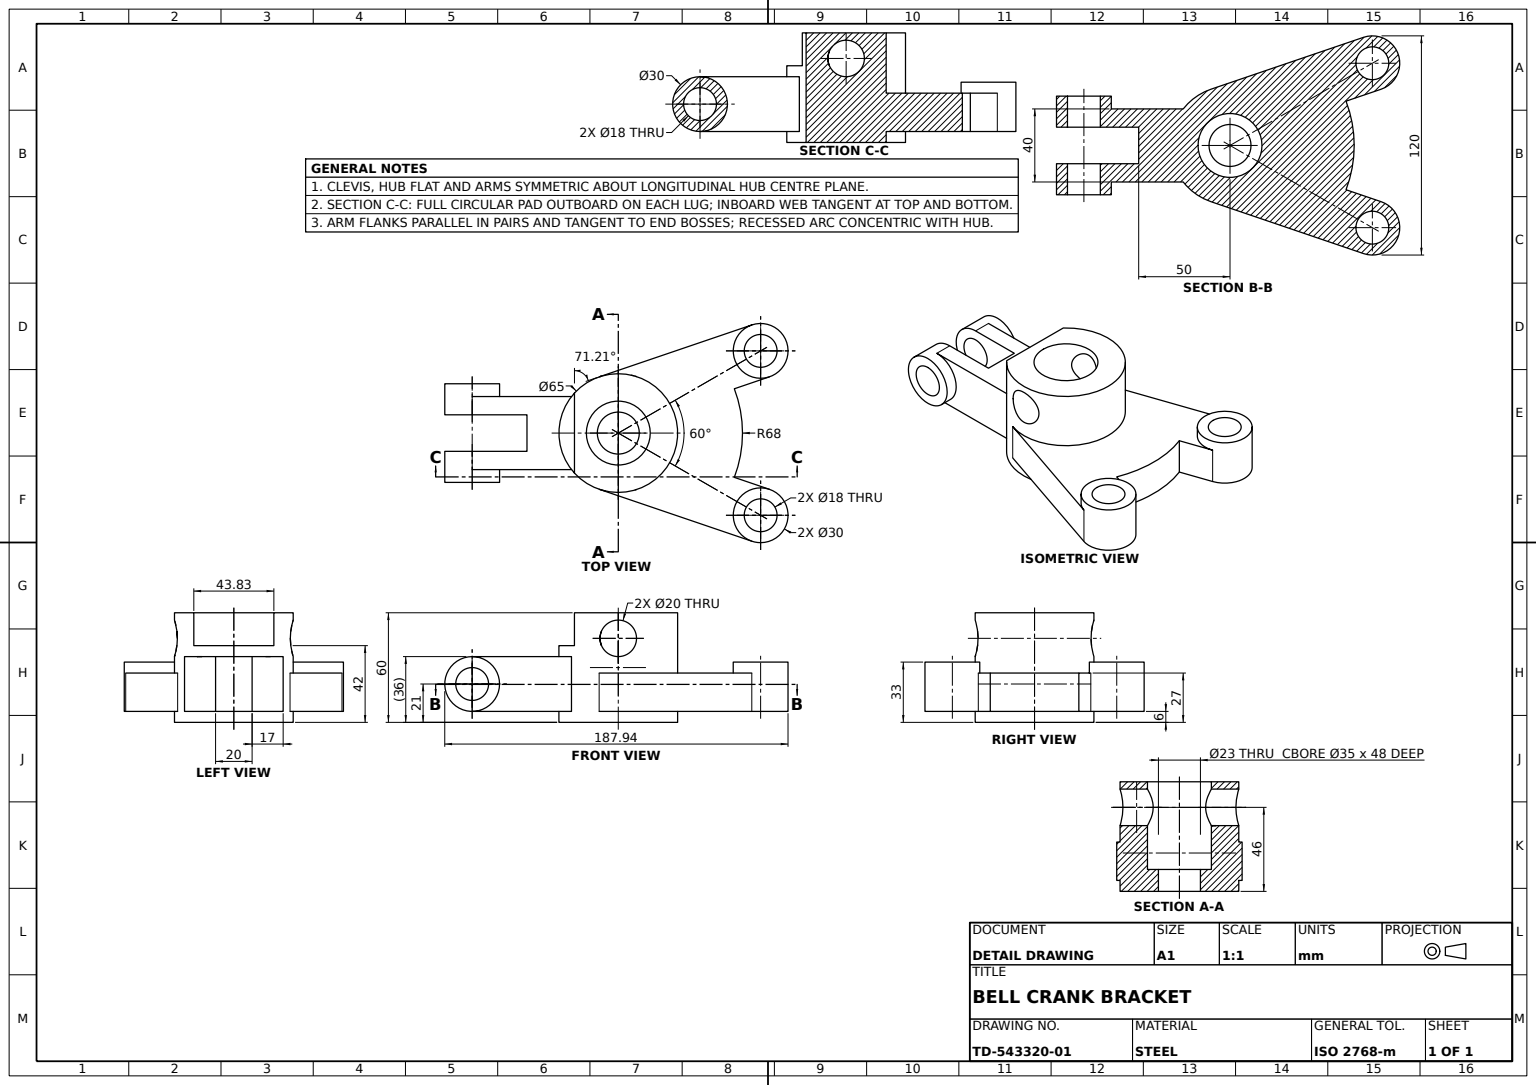
ISO-10303-21;
HEADER;
FILE_DESCRIPTION((''),'2;1');
FILE_NAME('','',(''),(''),'','','');
FILE_SCHEMA(('AUTOMOTIVE_DESIGN'));
ENDSEC;
DATA;
#1=APPLICATION_CONTEXT('');
#2=PRODUCT_CONTEXT('',#1,'mechanical');
#3=PRODUCT('','','',(#2));
#4=PRODUCT_DEFINITION_FORMATION('','',#3);
#5=PRODUCT_DEFINITION_CONTEXT('',#1,'design');
#6=PRODUCT_DEFINITION('','',#4,#5);
#7=PRODUCT_DEFINITION_SHAPE('','',#6);
#8=(LENGTH_UNIT()NAMED_UNIT(*)SI_UNIT(.MILLI.,.METRE.));
#9=(NAMED_UNIT(*)PLANE_ANGLE_UNIT()SI_UNIT($,.RADIAN.));
#10=(NAMED_UNIT(*)SI_UNIT($,.STERADIAN.)SOLID_ANGLE_UNIT());
#11=UNCERTAINTY_MEASURE_WITH_UNIT(LENGTH_MEASURE(0.005),#8,'distance_accuracy_value','');
#12=(GEOMETRIC_REPRESENTATION_CONTEXT(3)GLOBAL_UNCERTAINTY_ASSIGNED_CONTEXT((#11))GLOBAL_UNIT_ASSIGNED_CONTEXT((#8,#9,#10))REPRESENTATION_CONTEXT('',''));
#13=CARTESIAN_POINT('',(-80.,10.,6.));
#14=VERTEX_POINT('',#13);
#15=CARTESIAN_POINT('',(-80.,10.,36.));
#16=VERTEX_POINT('',#15);
#17=CARTESIAN_POINT('',(-80.,10.,21.));
#18=DIRECTION('',(0.,1.,0.));
#19=DIRECTION('',(-1.,0.,0.));
#20=AXIS2_PLACEMENT_3D('',#17,#18,#19);
#21=CIRCLE('',#20,15.);
#22=EDGE_CURVE('',#14,#16,#21,.T.);
#23=ORIENTED_EDGE('',*,*,#22,.T.);
#24=CARTESIAN_POINT('',(-80.,20.,36.));
#25=VERTEX_POINT('',#24);
#26=DIRECTION('',(0.,-1.,0.));
#27=VECTOR('',#26,1000.);
#28=LINE('',#24,#27);
#29=EDGE_CURVE('',#25,#16,#28,.T.);
#30=ORIENTED_EDGE('',*,*,#29,.F.);
#31=CARTESIAN_POINT('',(-80.,20.,6.));
#32=VERTEX_POINT('',#31);
#33=CARTESIAN_POINT('',(-80.,20.,21.));
#34=DIRECTION('',(1.,0.,0.));
#35=AXIS2_PLACEMENT_3D('',#33,#26,#34);
#36=CIRCLE('',#35,15.);
#37=EDGE_CURVE('',#25,#32,#36,.F.);
#38=ORIENTED_EDGE('',*,*,#37,.T.);
#39=LINE('',#31,#27);
#40=EDGE_CURVE('',#32,#14,#39,.T.);
#41=ORIENTED_EDGE('',*,*,#40,.T.);
#42=EDGE_LOOP('',(#23,#30,#38,#41));
#43=FACE_BOUND('',#42,.T.);
#44=CARTESIAN_POINT('',(-65.,27.,21.));
#45=VERTEX_POINT('',#44);
#46=CARTESIAN_POINT('',(-80.,27.,21.));
#47=AXIS2_PLACEMENT_3D('',#46,#26,#34);
#48=CIRCLE('',#47,15.);
#49=EDGE_CURVE('',#45,#45,#48,.T.);
#50=ORIENTED_EDGE('',*,*,#49,.T.);
#51=EDGE_LOOP('',(#50));
#52=FACE_BOUND('',#51,.T.);
#53=CARTESIAN_POINT('',(-80.,-27.,21.));
#54=DIRECTION('',(0.,0.,1.));
#55=AXIS2_PLACEMENT_3D('',#53,#18,#54);
#56=CYLINDRICAL_SURFACE('',#55,15.);
#57=ADVANCED_FACE('',(#43,#52),#56,.T.);
#58=CARTESIAN_POINT('',(-17.5,0.,60.));
#59=VERTEX_POINT('',#58);
#60=CARTESIAN_POINT('',(0.,0.,60.));
#61=DIRECTION('',(0.,0.,-1.));
#62=AXIS2_PLACEMENT_3D('',#60,#61,#19);
#63=CIRCLE('',#62,17.5);
#64=EDGE_CURVE('',#59,#59,#63,.T.);
#65=ORIENTED_EDGE('',*,*,#64,.F.);
#66=EDGE_LOOP('',(#65));
#67=FACE_BOUND('',#66,.T.);
#68=CARTESIAN_POINT('',(-17.5,0.,12.));
#69=VERTEX_POINT('',#68);
#70=CARTESIAN_POINT('',(0.,0.,12.));
#71=AXIS2_PLACEMENT_3D('',#70,#61,#19);
#72=CIRCLE('',#71,17.5);
#73=EDGE_CURVE('',#69,#69,#72,.F.);
#74=ORIENTED_EDGE('',*,*,#73,.F.);
#75=EDGE_LOOP('',(#74));
#76=FACE_BOUND('',#75,.T.);
#77=CARTESIAN_POINT('',(-10.,14.361407,46.));
#78=VERTEX_POINT('',#77);
#79=CARTESIAN_POINT('',(-9.438732,14.771794,41.979224));
#80=CARTESIAN_POINT('',(-10.279182,14.157174,46.004751));
#81=CARTESIAN_POINT('',(-9.444539,14.767949,50.001773));
#82=CARTESIAN_POINT('',(-7.260441,16.017563,53.224841));
#83=CARTESIAN_POINT('',(-4.030616,17.168631,55.434564));
#84=CARTESIAN_POINT('',(-0.036918,17.662745,56.277393));
#85=CARTESIAN_POINT('',(3.993432,17.180226,55.45558));
#86=CARTESIAN_POINT('',(7.242129,16.026003,53.242285));
#87=CARTESIAN_POINT('',(9.429111,14.778231,50.037006));
#88=CARTESIAN_POINT('',(10.279297,14.157085,46.035697));
#89=CARTESIAN_POINT('',(9.453393,14.762082,42.012147));
#90=CARTESIAN_POINT('',(7.268506,16.014082,38.783089));
#91=CARTESIAN_POINT('',(4.035859,17.167879,36.5664));
#92=CARTESIAN_POINT('',(0.033469,17.663376,35.721675));
#93=CARTESIAN_POINT('',(-4.002046,17.178482,36.547135));
#94=CARTESIAN_POINT('',(-7.252716,16.021359,38.768121));
#95=B_SPLINE_CURVE_WITH_KNOTS('',3,(#79,#80,#81,#82,#83,#84,#85,#86,#87,#88,#89,#90,#91,#92,#93,#94,#79,#80,#81),.UNSPECIFIED.,.T.,.F.,(1,1,1,1,1,1,1,1,1,1,1,1,1,1,1,1,1,1,1,1,1,1,1),(-0.011982501,-0.007988334,-0.003994167,0.,0.003994167,0.007988334,0.011982501,0.015976668,0.019970836,0.023965003,0.02795917,0.031953337,0.035947504,0.039941671,0.043935838,0.047930005,0.051924173,0.05591834,0.059912507,0.063906674,0.067900841,0.071895008,0.075889175),.UNSPECIFIED.);
#96=EDGE_CURVE('',#78,#78,#95,.T.);
#97=ORIENTED_EDGE('',*,*,#96,.T.);
#98=EDGE_LOOP('',(#97));
#99=FACE_BOUND('',#98,.T.);
#100=CARTESIAN_POINT('',(-10.,-14.361407,46.));
#101=VERTEX_POINT('',#100);
#102=CARTESIAN_POINT('',(-9.438732,-14.771794,50.020776));
#103=CARTESIAN_POINT('',(-10.279182,-14.157174,45.995249));
#104=CARTESIAN_POINT('',(-9.444539,-14.767949,41.998227));
#105=CARTESIAN_POINT('',(-7.260441,-16.017563,38.775159));
#106=CARTESIAN_POINT('',(-4.030616,-17.168631,36.565436));
#107=CARTESIAN_POINT('',(-0.036918,-17.662745,35.722607));
#108=CARTESIAN_POINT('',(3.993432,-17.180226,36.54442));
#109=CARTESIAN_POINT('',(7.242129,-16.026003,38.757715));
#110=CARTESIAN_POINT('',(9.429111,-14.778231,41.962994));
#111=CARTESIAN_POINT('',(10.279297,-14.157085,45.964303));
#112=CARTESIAN_POINT('',(9.453393,-14.762082,49.987853));
#113=CARTESIAN_POINT('',(7.268506,-16.014082,53.216911));
#114=CARTESIAN_POINT('',(4.035859,-17.167879,55.4336));
#115=CARTESIAN_POINT('',(0.033469,-17.663376,56.278325));
#116=CARTESIAN_POINT('',(-4.002046,-17.178482,55.452865));
#117=CARTESIAN_POINT('',(-7.252716,-16.021359,53.231879));
#118=B_SPLINE_CURVE_WITH_KNOTS('',3,(#102,#103,#104,#105,#106,#107,#108,#109,#110,#111,#112,#113,#114,#115,#116,#117,#102,#103,#104),.UNSPECIFIED.,.T.,.F.,(1,1,1,1,1,1,1,1,1,1,1,1,1,1,1,1,1,1,1,1,1,1,1),(-0.011982501,-0.007988334,-0.003994167,0.,0.003994167,0.007988334,0.011982501,0.015976668,0.019970836,0.023965003,0.02795917,0.031953337,0.035947504,0.039941671,0.043935838,0.047930005,0.051924173,0.05591834,0.059912507,0.063906674,0.067900841,0.071895008,0.075889175),.UNSPECIFIED.);
#119=EDGE_CURVE('',#101,#101,#118,.T.);
#120=ORIENTED_EDGE('',*,*,#119,.T.);
#121=EDGE_LOOP('',(#120));
#122=FACE_BOUND('',#121,.T.);
#123=CYLINDRICAL_SURFACE('',#62,17.5);
#124=ADVANCED_FACE('',(#67,#76,#99,#122),#123,.F.);
#125=CARTESIAN_POINT('',(82.77323,-30.799226,27.));
#126=VERTEX_POINT('',#125);
#127=CARTESIAN_POINT('',(82.77323,-30.799226,6.));
#128=VERTEX_POINT('',#127);
#129=VECTOR('',#61,1000.);
#130=LINE('',#125,#129);
#131=EDGE_CURVE('',#126,#128,#130,.T.);
#132=ORIENTED_EDGE('',*,*,#131,.T.);
#133=CARTESIAN_POINT('',(63.528162,-24.25227,6.));
#134=VERTEX_POINT('',#133);
#135=DIRECTION('',(0.94671826,-0.322062938,0.));
#136=VECTOR('',#135,1000.);
#137=LINE('',#133,#136);
#138=EDGE_CURVE('',#134,#128,#137,.T.);
#139=ORIENTED_EDGE('',*,*,#138,.F.);
#140=CARTESIAN_POINT('',(63.528162,-24.25227,27.));
#141=VERTEX_POINT('',#140);
#142=LINE('',#140,#129);
#143=EDGE_CURVE('',#134,#141,#142,.F.);
#144=ORIENTED_EDGE('',*,*,#143,.T.);
#145=LINE('',#140,#136);
#146=EDGE_CURVE('',#141,#126,#145,.T.);
#147=ORIENTED_EDGE('',*,*,#146,.T.);
#148=EDGE_LOOP('',(#132,#139,#144,#147));
#149=FACE_BOUND('',#148,.T.);
#150=DIRECTION('',(0.322062938,0.94671826,0.));
#151=DIRECTION('',(-0.94671826,0.322062938,0.));
#152=AXIS2_PLACEMENT_3D('',#140,#150,#151);
#153=PLANE('',#152);
#154=ADVANCED_FACE('',(#149),#153,.T.);
#155=CARTESIAN_POINT('',(-80.,-20.,6.));
#156=VERTEX_POINT('',#155);
#157=CARTESIAN_POINT('',(-25.617377,-20.,6.));
#158=VERTEX_POINT('',#157);
#159=VECTOR('',#34,1000.);
#160=LINE('',#155,#159);
#161=EDGE_CURVE('',#156,#158,#160,.T.);
#162=ORIENTED_EDGE('',*,*,#161,.T.);
#163=CARTESIAN_POINT('',(-25.617377,-20.,36.));
#164=VERTEX_POINT('',#163);
#165=CARTESIAN_POINT('',(-25.617377,-20.,60.));
#166=LINE('',#165,#129);
#167=EDGE_CURVE('',#164,#158,#166,.T.);
#168=ORIENTED_EDGE('',*,*,#167,.F.);
#169=CARTESIAN_POINT('',(-80.,-20.,36.));
#170=VERTEX_POINT('',#169);
#171=LINE('',#169,#159);
#172=EDGE_CURVE('',#170,#164,#171,.T.);
#173=ORIENTED_EDGE('',*,*,#172,.F.);
#174=CARTESIAN_POINT('',(-80.,-20.,21.));
#175=AXIS2_PLACEMENT_3D('',#174,#18,#19);
#176=CIRCLE('',#175,15.);
#177=EDGE_CURVE('',#156,#170,#176,.F.);
#178=ORIENTED_EDGE('',*,*,#177,.F.);
#179=EDGE_LOOP('',(#162,#168,#173,#178));
#180=FACE_BOUND('',#179,.T.);
#181=AXIS2_PLACEMENT_3D('',#169,#18,#19);
#182=PLANE('',#181);
#183=ADVANCED_FACE('',(#180),#182,.F.);
#184=CARTESIAN_POINT('',(63.528162,24.25227,27.));
#185=VERTEX_POINT('',#184);
#186=CARTESIAN_POINT('',(0.,0.,27.));
#187=AXIS2_PLACEMENT_3D('',#186,#61,#26);
#188=CIRCLE('',#187,68.);
#189=EDGE_CURVE('',#185,#141,#188,.T.);
#190=ORIENTED_EDGE('',*,*,#189,.T.);
#191=ORIENTED_EDGE('',*,*,#143,.F.);
#192=CARTESIAN_POINT('',(63.528162,24.25227,6.));
#193=VERTEX_POINT('',#192);
#194=CARTESIAN_POINT('',(0.,0.,6.));
#195=AXIS2_PLACEMENT_3D('',#194,#61,#26);
#196=CIRCLE('',#195,68.);
#197=EDGE_CURVE('',#193,#134,#196,.T.);
#198=ORIENTED_EDGE('',*,*,#197,.F.);
#199=LINE('',#184,#129);
#200=EDGE_CURVE('',#193,#185,#199,.F.);
#201=ORIENTED_EDGE('',*,*,#200,.T.);
#202=EDGE_LOOP('',(#190,#191,#198,#201));
#203=FACE_BOUND('',#202,.T.);
#204=AXIS2_PLACEMENT_3D('',#186,#61,#19);
#205=CYLINDRICAL_SURFACE('',#204,68.);
#206=ADVANCED_FACE('',(#203),#205,.T.);
#207=CARTESIAN_POINT('',(-10.,30.923292,46.));
#208=VERTEX_POINT('',#207);
#209=CARTESIAN_POINT('',(-9.466897,31.102927,42.04327));
#210=CARTESIAN_POINT('',(-10.266055,30.833623,46.001431));
#211=CARTESIAN_POINT('',(-9.468882,31.102334,49.951005));
#212=CARTESIAN_POINT('',(-7.250854,31.724092,53.252689));
#213=CARTESIAN_POINT('',(-3.950054,32.330867,55.468701));
#214=CARTESIAN_POINT('',(-0.008238,32.584227,56.264458));
#215=CARTESIAN_POINT('',(3.943691,32.33222,55.473454));
#216=CARTESIAN_POINT('',(7.255547,31.723107,53.249164));
#217=CARTESIAN_POINT('',(9.469782,31.10195,49.947041));
#218=CARTESIAN_POINT('',(10.264312,30.834201,46.005071));
#219=CARTESIAN_POINT('',(9.472964,31.101,42.058399));
#220=CARTESIAN_POINT('',(7.256614,31.722822,38.752123));
#221=CARTESIAN_POINT('',(3.950668,32.331094,36.530395));
#222=CARTESIAN_POINT('',(0.002274,32.584319,35.735284));
#223=CARTESIAN_POINT('',(-3.946024,32.331631,36.528469));
#224=CARTESIAN_POINT('',(-7.250616,31.72414,38.747709));
#225=B_SPLINE_CURVE_WITH_KNOTS('',3,(#209,#210,#211,#212,#213,#214,#215,#216,#217,#218,#219,#220,#221,#222,#223,#224,#209,#210,#211),.UNSPECIFIED.,.T.,.F.,(1,1,1,1,1,1,1,1,1,1,1,1,1,1,1,1,1,1,1,1,1,1,1),(-0.011794379,-0.007862919,-0.00393146,0.,0.00393146,0.007862919,0.011794379,0.015725838,0.019657298,0.023588757,0.027520217,0.031451676,0.035383136,0.039314595,0.043246055,0.047177514,0.051108974,0.055040433,0.058971893,0.062903352,0.066834812,0.070766271,0.074697731),.UNSPECIFIED.);
#226=EDGE_CURVE('',#208,#208,#225,.T.);
#227=ORIENTED_EDGE('',*,*,#226,.F.);
#228=EDGE_LOOP('',(#227));
#229=FACE_BOUND('',#228,.T.);
#230=CARTESIAN_POINT('',(-10.,-30.923292,46.));
#231=VERTEX_POINT('',#230);
#232=CARTESIAN_POINT('',(-9.466897,-31.102927,49.95673));
#233=CARTESIAN_POINT('',(-10.266055,-30.833623,45.998569));
#234=CARTESIAN_POINT('',(-9.468882,-31.102334,42.048995));
#235=CARTESIAN_POINT('',(-7.250854,-31.724092,38.747311));
#236=CARTESIAN_POINT('',(-3.950054,-32.330867,36.531299));
#237=CARTESIAN_POINT('',(-0.008238,-32.584227,35.735542));
#238=CARTESIAN_POINT('',(3.943691,-32.33222,36.526546));
#239=CARTESIAN_POINT('',(7.255547,-31.723107,38.750836));
#240=CARTESIAN_POINT('',(9.469782,-31.10195,42.052959));
#241=CARTESIAN_POINT('',(10.264312,-30.834201,45.994929));
#242=CARTESIAN_POINT('',(9.472964,-31.101,49.941601));
#243=CARTESIAN_POINT('',(7.256614,-31.722822,53.247877));
#244=CARTESIAN_POINT('',(3.950668,-32.331094,55.469605));
#245=CARTESIAN_POINT('',(0.002274,-32.584319,56.264716));
#246=CARTESIAN_POINT('',(-3.946024,-32.331631,55.471531));
#247=CARTESIAN_POINT('',(-7.250616,-31.72414,53.252291));
#248=B_SPLINE_CURVE_WITH_KNOTS('',3,(#232,#233,#234,#235,#236,#237,#238,#239,#240,#241,#242,#243,#244,#245,#246,#247,#232,#233,#234),.UNSPECIFIED.,.T.,.F.,(1,1,1,1,1,1,1,1,1,1,1,1,1,1,1,1,1,1,1,1,1,1,1),(-0.011794379,-0.007862919,-0.00393146,0.,0.00393146,0.007862919,0.011794379,0.015725838,0.019657298,0.023588757,0.027520217,0.031451676,0.035383136,0.039314595,0.043246055,0.047177514,0.051108974,0.055040433,0.058971893,0.062903352,0.066834812,0.070766271,0.074697731),.UNSPECIFIED.);
#249=EDGE_CURVE('',#231,#231,#248,.T.);
#250=ORIENTED_EDGE('',*,*,#249,.F.);
#251=EDGE_LOOP('',(#250));
#252=FACE_BOUND('',#251,.T.);
#253=CARTESIAN_POINT('',(32.5,0.,0.));
#254=VERTEX_POINT('',#253);
#255=CARTESIAN_POINT('',(0.,0.,0.));
#256=AXIS2_PLACEMENT_3D('',#255,#61,#34);
#257=CIRCLE('',#256,32.5);
#258=EDGE_CURVE('',#254,#254,#257,.T.);
#259=ORIENTED_EDGE('',*,*,#258,.F.);
#260=EDGE_LOOP('',(#259));
#261=FACE_BOUND('',#260,.T.);
#262=CARTESIAN_POINT('',(-24.,-21.914607,42.));
#263=VERTEX_POINT('',#262);
#264=CARTESIAN_POINT('',(-24.,-21.914607,60.));
#265=VERTEX_POINT('',#264);
#266=LINE('',#264,#129);
#267=EDGE_CURVE('',#263,#265,#266,.F.);
#268=ORIENTED_EDGE('',*,*,#267,.F.);
#269=CARTESIAN_POINT('',(-24.,21.914607,42.));
#270=VERTEX_POINT('',#269);
#271=CARTESIAN_POINT('',(0.,0.,42.));
#272=AXIS2_PLACEMENT_3D('',#271,#61,#19);
#273=CIRCLE('',#272,32.5);
#274=EDGE_CURVE('',#270,#263,#273,.F.);
#275=ORIENTED_EDGE('',*,*,#274,.F.);
#276=CARTESIAN_POINT('',(-24.,21.914607,60.));
#277=VERTEX_POINT('',#276);
#278=LINE('',#276,#129);
#279=EDGE_CURVE('',#277,#270,#278,.T.);
#280=ORIENTED_EDGE('',*,*,#279,.F.);
#281=AXIS2_PLACEMENT_3D('',#60,#61,#34);
#282=CIRCLE('',#281,32.5);
#283=EDGE_CURVE('',#277,#265,#282,.T.);
#284=ORIENTED_EDGE('',*,*,#283,.T.);
#285=EDGE_LOOP('',(#268,#275,#280,#284));
#286=FACE_BOUND('',#285,.T.);
#287=CARTESIAN_POINT('',(-10.467045,-30.768343,6.));
#288=VERTEX_POINT('',#287);
#289=CARTESIAN_POINT('',(-10.467045,30.768343,6.));
#290=VERTEX_POINT('',#289);
#291=AXIS2_PLACEMENT_3D('',#194,#61,#19);
#292=CIRCLE('',#291,32.5);
#293=EDGE_CURVE('',#288,#290,#292,.F.);
#294=ORIENTED_EDGE('',*,*,#293,.F.);
#295=CARTESIAN_POINT('',(-10.467045,-30.768343,27.));
#296=VERTEX_POINT('',#295);
#297=LINE('',#295,#129);
#298=EDGE_CURVE('',#296,#288,#297,.T.);
#299=ORIENTED_EDGE('',*,*,#298,.F.);
#300=CARTESIAN_POINT('',(-10.467045,30.768343,27.));
#301=VERTEX_POINT('',#300);
#302=CIRCLE('',#204,32.5);
#303=EDGE_CURVE('',#296,#301,#302,.F.);
#304=ORIENTED_EDGE('',*,*,#303,.T.);
#305=LINE('',#300,#129);
#306=EDGE_CURVE('',#301,#290,#305,.T.);
#307=ORIENTED_EDGE('',*,*,#306,.T.);
#308=EDGE_LOOP('',(#294,#299,#304,#307));
#309=FACE_BOUND('',#308,.T.);
#310=ORIENTED_EDGE('',*,*,#167,.T.);
#311=CARTESIAN_POINT('',(-25.617377,20.,6.));
#312=VERTEX_POINT('',#311);
#313=AXIS2_PLACEMENT_3D('',#194,#54,#34);
#314=CIRCLE('',#313,32.5);
#315=EDGE_CURVE('',#158,#312,#314,.F.);
#316=ORIENTED_EDGE('',*,*,#315,.T.);
#317=CARTESIAN_POINT('',(-25.617377,20.,36.));
#318=VERTEX_POINT('',#317);
#319=CARTESIAN_POINT('',(-25.617377,20.,60.));
#320=LINE('',#319,#129);
#321=EDGE_CURVE('',#312,#318,#320,.F.);
#322=ORIENTED_EDGE('',*,*,#321,.T.);
#323=CARTESIAN_POINT('',(0.,0.,36.));
#324=AXIS2_PLACEMENT_3D('',#323,#54,#34);
#325=CIRCLE('',#324,32.5);
#326=EDGE_CURVE('',#164,#318,#325,.F.);
#327=ORIENTED_EDGE('',*,*,#326,.F.);
#328=EDGE_LOOP('',(#310,#316,#322,#327));
#329=FACE_BOUND('',#328,.T.);
#330=CYLINDRICAL_SURFACE('',#62,32.5);
#331=ADVANCED_FACE('',(#229,#252,#261,#286,#309,#329),#330,.T.);
#332=ORIENTED_EDGE('',*,*,#37,.F.);
#333=CARTESIAN_POINT('',(-20.,20.,36.));
#334=VECTOR('',#19,1000.);
#335=LINE('',#333,#334);
#336=EDGE_CURVE('',#318,#25,#335,.T.);
#337=ORIENTED_EDGE('',*,*,#336,.F.);
#338=ORIENTED_EDGE('',*,*,#321,.F.);
#339=CARTESIAN_POINT('',(-20.,20.,6.));
#340=LINE('',#339,#334);
#341=EDGE_CURVE('',#312,#32,#340,.T.);
#342=ORIENTED_EDGE('',*,*,#341,.T.);
#343=EDGE_LOOP('',(#332,#337,#338,#342));
#344=FACE_BOUND('',#343,.T.);
#345=AXIS2_PLACEMENT_3D('',#333,#26,#34);
#346=PLANE('',#345);
#347=ADVANCED_FACE('',(#344),#346,.F.);
#348=CARTESIAN_POINT('',(82.77323,30.799226,27.));
#349=VERTEX_POINT('',#348);
#350=DIRECTION('',(-0.94671826,-0.322062938,0.));
#351=VECTOR('',#350,1000.);
#352=LINE('',#348,#351);
#353=EDGE_CURVE('',#349,#185,#352,.T.);
#354=ORIENTED_EDGE('',*,*,#353,.T.);
#355=ORIENTED_EDGE('',*,*,#200,.F.);
#356=CARTESIAN_POINT('',(82.77323,30.799226,6.));
#357=VERTEX_POINT('',#356);
#358=LINE('',#356,#351);
#359=EDGE_CURVE('',#357,#193,#358,.T.);
#360=ORIENTED_EDGE('',*,*,#359,.F.);
#361=LINE('',#348,#129);
#362=EDGE_CURVE('',#349,#357,#361,.T.);
#363=ORIENTED_EDGE('',*,*,#362,.F.);
#364=EDGE_LOOP('',(#354,#355,#360,#363));
#365=FACE_BOUND('',#364,.T.);
#366=DIRECTION('',(0.322062938,-0.94671826,0.));
#367=DIRECTION('',(0.94671826,0.322062938,0.));
#368=AXIS2_PLACEMENT_3D('',#348,#366,#367);
#369=PLANE('',#368);
#370=ADVANCED_FACE('',(#365),#369,.T.);
#371=ORIENTED_EDGE('',*,*,#96,.F.);
#372=EDGE_LOOP('',(#371));
#373=FACE_BOUND('',#372,.T.);
#374=ORIENTED_EDGE('',*,*,#226,.T.);
#375=EDGE_LOOP('',(#374));
#376=FACE_BOUND('',#375,.T.);
#377=CARTESIAN_POINT('',(0.,-32.5,46.));
#378=AXIS2_PLACEMENT_3D('',#377,#18,#19);
#379=CYLINDRICAL_SURFACE('',#378,10.);
#380=ADVANCED_FACE('',(#373,#376),#379,.F.);
#381=CARTESIAN_POINT('',(-24.,0.,60.));
#382=LINE('',#381,#27);
#383=EDGE_CURVE('',#277,#265,#382,.T.);
#384=ORIENTED_EDGE('',*,*,#383,.F.);
#385=ORIENTED_EDGE('',*,*,#279,.T.);
#386=CARTESIAN_POINT('',(-24.,-55.,42.));
#387=VECTOR('',#18,1000.);
#388=LINE('',#386,#387);
#389=EDGE_CURVE('',#270,#263,#388,.F.);
#390=ORIENTED_EDGE('',*,*,#389,.T.);
#391=ORIENTED_EDGE('',*,*,#267,.T.);
#392=EDGE_LOOP('',(#384,#385,#390,#391));
#393=FACE_BOUND('',#392,.T.);
#394=CARTESIAN_POINT('',(-24.,-55.,70.));
#395=AXIS2_PLACEMENT_3D('',#394,#34,#61);
#396=PLANE('',#395);
#397=ADVANCED_FACE('',(#393),#396,.F.);
#398=CARTESIAN_POINT('',(77.942286,30.,33.));
#399=VERTEX_POINT('',#398);
#400=CARTESIAN_POINT('',(77.942286,45.,33.));
#401=AXIS2_PLACEMENT_3D('',#400,#54,#26);
#402=CIRCLE('',#401,15.);
#403=EDGE_CURVE('',#399,#399,#402,.T.);
#404=ORIENTED_EDGE('',*,*,#403,.F.);
#405=EDGE_LOOP('',(#404));
#406=FACE_BOUND('',#405,.T.);
#407=CARTESIAN_POINT('',(73.111342,59.200774,27.));
#408=VERTEX_POINT('',#407);
#409=CARTESIAN_POINT('',(73.111342,59.200774,6.));
#410=VERTEX_POINT('',#409);
#411=LINE('',#407,#129);
#412=EDGE_CURVE('',#408,#410,#411,.T.);
#413=ORIENTED_EDGE('',*,*,#412,.F.);
#414=CARTESIAN_POINT('',(77.942286,45.,27.));
#415=AXIS2_PLACEMENT_3D('',#414,#61,#19);
#416=CIRCLE('',#415,15.);
#417=EDGE_CURVE('',#408,#349,#416,.F.);
#418=ORIENTED_EDGE('',*,*,#417,.T.);
#419=ORIENTED_EDGE('',*,*,#362,.T.);
#420=CARTESIAN_POINT('',(77.942286,45.,6.));
#421=AXIS2_PLACEMENT_3D('',#420,#61,#26);
#422=CIRCLE('',#421,15.);
#423=EDGE_CURVE('',#410,#357,#422,.T.);
#424=ORIENTED_EDGE('',*,*,#423,.F.);
#425=EDGE_LOOP('',(#413,#418,#419,#424));
#426=FACE_BOUND('',#425,.T.);
#427=CYLINDRICAL_SURFACE('',#415,15.);
#428=ADVANCED_FACE('',(#406,#426),#427,.T.);
#429=ORIENTED_EDGE('',*,*,#64,.T.);
#430=EDGE_LOOP('',(#429));
#431=FACE_BOUND('',#430,.T.);
#432=ORIENTED_EDGE('',*,*,#283,.F.);
#433=ORIENTED_EDGE('',*,*,#383,.T.);
#434=EDGE_LOOP('',(#432,#433));
#435=FACE_BOUND('',#434,.T.);
#436=PLANE('',#62);
#437=ADVANCED_FACE('',(#431,#435),#436,.F.);
#438=ORIENTED_EDGE('',*,*,#326,.T.);
#439=ORIENTED_EDGE('',*,*,#336,.T.);
#440=ORIENTED_EDGE('',*,*,#29,.T.);
#441=CARTESIAN_POINT('',(-50.,10.,36.));
#442=VERTEX_POINT('',#441);
#443=CARTESIAN_POINT('',(0.,10.,36.));
#444=LINE('',#443,#334);
#445=EDGE_CURVE('',#442,#16,#444,.T.);
#446=ORIENTED_EDGE('',*,*,#445,.F.);
#447=CARTESIAN_POINT('',(-50.,-10.,36.));
#448=VERTEX_POINT('',#447);
#449=CARTESIAN_POINT('',(-50.,0.,36.));
#450=LINE('',#449,#387);
#451=EDGE_CURVE('',#448,#442,#450,.T.);
#452=ORIENTED_EDGE('',*,*,#451,.F.);
#453=CARTESIAN_POINT('',(-80.,-10.,36.));
#454=VERTEX_POINT('',#453);
#455=CARTESIAN_POINT('',(0.,-10.,36.));
#456=LINE('',#455,#159);
#457=EDGE_CURVE('',#454,#448,#456,.T.);
#458=ORIENTED_EDGE('',*,*,#457,.F.);
#459=EDGE_CURVE('',#454,#170,#28,.T.);
#460=ORIENTED_EDGE('',*,*,#459,.T.);
#461=ORIENTED_EDGE('',*,*,#172,.T.);
#462=EDGE_LOOP('',(#438,#439,#440,#446,#452,#458,#460,#461));
#463=FACE_BOUND('',#462,.T.);
#464=PLANE('',#324);
#465=ADVANCED_FACE('',(#463),#464,.T.);
#466=ORIENTED_EDGE('',*,*,#177,.T.);
#467=ORIENTED_EDGE('',*,*,#459,.F.);
#468=CARTESIAN_POINT('',(-80.,-10.,6.));
#469=VERTEX_POINT('',#468);
#470=CARTESIAN_POINT('',(-80.,-10.,21.));
#471=AXIS2_PLACEMENT_3D('',#470,#26,#34);
#472=CIRCLE('',#471,15.);
#473=EDGE_CURVE('',#454,#469,#472,.T.);
#474=ORIENTED_EDGE('',*,*,#473,.T.);
#475=EDGE_CURVE('',#469,#156,#39,.T.);
#476=ORIENTED_EDGE('',*,*,#475,.T.);
#477=EDGE_LOOP('',(#466,#467,#474,#476));
#478=FACE_BOUND('',#477,.T.);
#479=CARTESIAN_POINT('',(-65.,-27.,21.));
#480=VERTEX_POINT('',#479);
#481=AXIS2_PLACEMENT_3D('',#53,#26,#34);
#482=CIRCLE('',#481,15.);
#483=EDGE_CURVE('',#480,#480,#482,.T.);
#484=ORIENTED_EDGE('',*,*,#483,.F.);
#485=EDGE_LOOP('',(#484));
#486=FACE_BOUND('',#485,.T.);
#487=ADVANCED_FACE('',(#478,#486),#56,.T.);
#488=ORIENTED_EDGE('',*,*,#403,.T.);
#489=EDGE_LOOP('',(#488));
#490=FACE_BOUND('',#489,.T.);
#491=CARTESIAN_POINT('',(68.942286,45.,33.));
#492=VERTEX_POINT('',#491);
#493=AXIS2_PLACEMENT_3D('',#400,#61,#19);
#494=CIRCLE('',#493,9.);
#495=EDGE_CURVE('',#492,#492,#494,.T.);
#496=ORIENTED_EDGE('',*,*,#495,.T.);
#497=EDGE_LOOP('',(#496));
#498=FACE_BOUND('',#497,.T.);
#499=AXIS2_PLACEMENT_3D('',#400,#54,#34);
#500=PLANE('',#499);
#501=ADVANCED_FACE('',(#490,#498),#500,.T.);
#502=ORIENTED_EDGE('',*,*,#258,.T.);
#503=EDGE_LOOP('',(#502));
#504=FACE_BOUND('',#503,.T.);
#505=CARTESIAN_POINT('',(-11.5,0.,0.));
#506=VERTEX_POINT('',#505);
#507=AXIS2_PLACEMENT_3D('',#255,#61,#19);
#508=CIRCLE('',#507,11.5);
#509=EDGE_CURVE('',#506,#506,#508,.T.);
#510=ORIENTED_EDGE('',*,*,#509,.F.);
#511=EDGE_LOOP('',(#510));
#512=FACE_BOUND('',#511,.T.);
#513=PLANE('',#507);
#514=ADVANCED_FACE('',(#504,#512),#513,.T.);
#515=ORIENTED_EDGE('',*,*,#509,.T.);
#516=EDGE_LOOP('',(#515));
#517=FACE_BOUND('',#516,.T.);
#518=CARTESIAN_POINT('',(-11.5,0.,12.));
#519=VERTEX_POINT('',#518);
#520=CIRCLE('',#71,11.5);
#521=EDGE_CURVE('',#519,#519,#520,.F.);
#522=ORIENTED_EDGE('',*,*,#521,.T.);
#523=EDGE_LOOP('',(#522));
#524=FACE_BOUND('',#523,.T.);
#525=CARTESIAN_POINT('',(0.,0.,-96.999756));
#526=AXIS2_PLACEMENT_3D('',#525,#61,#19);
#527=CYLINDRICAL_SURFACE('',#526,11.5);
#528=ADVANCED_FACE('',(#517,#524),#527,.F.);
#529=VECTOR('',#367,1000.);
#530=LINE('',#289,#529);
#531=EDGE_CURVE('',#290,#410,#530,.T.);
#532=ORIENTED_EDGE('',*,*,#531,.F.);
#533=ORIENTED_EDGE('',*,*,#306,.F.);
#534=LINE('',#300,#529);
#535=EDGE_CURVE('',#301,#408,#534,.T.);
#536=ORIENTED_EDGE('',*,*,#535,.T.);
#537=ORIENTED_EDGE('',*,*,#412,.T.);
#538=EDGE_LOOP('',(#532,#533,#536,#537));
#539=FACE_BOUND('',#538,.T.);
#540=DIRECTION('',(-0.322062938,0.94671826,0.));
#541=AXIS2_PLACEMENT_3D('',#300,#540,#350);
#542=PLANE('',#541);
#543=ADVANCED_FACE('',(#539),#542,.T.);
#544=CARTESIAN_POINT('',(-80.,27.,12.));
#545=VERTEX_POINT('',#544);
#546=AXIS2_PLACEMENT_3D('',#46,#26,#61);
#547=CIRCLE('',#546,9.);
#548=EDGE_CURVE('',#545,#545,#547,.T.);
#549=ORIENTED_EDGE('',*,*,#548,.T.);
#550=EDGE_LOOP('',(#549));
#551=FACE_BOUND('',#550,.T.);
#552=ORIENTED_EDGE('',*,*,#49,.F.);
#553=EDGE_LOOP('',(#552));
#554=FACE_BOUND('',#553,.T.);
#555=PLANE('',#546);
#556=ADVANCED_FACE('',(#551,#554),#555,.F.);
#557=CARTESIAN_POINT('',(-50.,10.,6.));
#558=VERTEX_POINT('',#557);
#559=CARTESIAN_POINT('',(-50.,10.,55.));
#560=LINE('',#559,#129);
#561=EDGE_CURVE('',#558,#442,#560,.F.);
#562=ORIENTED_EDGE('',*,*,#561,.T.);
#563=ORIENTED_EDGE('',*,*,#445,.T.);
#564=ORIENTED_EDGE('',*,*,#22,.F.);
#565=CARTESIAN_POINT('',(0.,10.,6.));
#566=LINE('',#565,#334);
#567=EDGE_CURVE('',#558,#14,#566,.T.);
#568=ORIENTED_EDGE('',*,*,#567,.F.);
#569=EDGE_LOOP('',(#562,#563,#564,#568));
#570=FACE_BOUND('',#569,.T.);
#571=CARTESIAN_POINT('',(-89.,10.,21.));
#572=VERTEX_POINT('',#571);
#573=CIRCLE('',#20,9.);
#574=EDGE_CURVE('',#572,#572,#573,.T.);
#575=ORIENTED_EDGE('',*,*,#574,.T.);
#576=EDGE_LOOP('',(#575));
#577=FACE_BOUND('',#576,.T.);
#578=CARTESIAN_POINT('',(-102.395946,10.,55.));
#579=AXIS2_PLACEMENT_3D('',#578,#18,#19);
#580=PLANE('',#579);
#581=ADVANCED_FACE('',(#570,#577),#580,.F.);
#582=ORIENTED_EDGE('',*,*,#119,.F.);
#583=EDGE_LOOP('',(#582));
#584=FACE_BOUND('',#583,.T.);
#585=ORIENTED_EDGE('',*,*,#249,.T.);
#586=EDGE_LOOP('',(#585));
#587=FACE_BOUND('',#586,.T.);
#588=ADVANCED_FACE('',(#584,#587),#379,.F.);
#589=ORIENTED_EDGE('',*,*,#574,.F.);
#590=EDGE_LOOP('',(#589));
#591=FACE_BOUND('',#590,.T.);
#592=ORIENTED_EDGE('',*,*,#548,.F.);
#593=EDGE_LOOP('',(#592));
#594=FACE_BOUND('',#593,.T.);
#595=CYLINDRICAL_SURFACE('',#55,9.);
#596=ADVANCED_FACE('',(#591,#594),#595,.F.);
#597=CARTESIAN_POINT('',(-71.,-10.,21.));
#598=VERTEX_POINT('',#597);
#599=CIRCLE('',#471,9.);
#600=EDGE_CURVE('',#598,#598,#599,.T.);
#601=ORIENTED_EDGE('',*,*,#600,.F.);
#602=EDGE_LOOP('',(#601));
#603=FACE_BOUND('',#602,.T.);
#604=CARTESIAN_POINT('',(-80.,-27.,30.));
#605=VERTEX_POINT('',#604);
#606=CIRCLE('',#55,9.);
#607=EDGE_CURVE('',#605,#605,#606,.T.);
#608=ORIENTED_EDGE('',*,*,#607,.F.);
#609=EDGE_LOOP('',(#608));
#610=FACE_BOUND('',#609,.T.);
#611=ADVANCED_FACE('',(#603,#610),#595,.F.);
#612=CARTESIAN_POINT('',(73.111342,-59.200774,27.));
#613=VERTEX_POINT('',#612);
#614=CARTESIAN_POINT('',(73.111342,-59.200774,6.));
#615=VERTEX_POINT('',#614);
#616=LINE('',#612,#129);
#617=EDGE_CURVE('',#613,#615,#616,.T.);
#618=ORIENTED_EDGE('',*,*,#617,.T.);
#619=CARTESIAN_POINT('',(77.942286,-45.,6.));
#620=AXIS2_PLACEMENT_3D('',#619,#61,#26);
#621=CIRCLE('',#620,15.);
#622=EDGE_CURVE('',#128,#615,#621,.T.);
#623=ORIENTED_EDGE('',*,*,#622,.F.);
#624=ORIENTED_EDGE('',*,*,#131,.F.);
#625=CARTESIAN_POINT('',(77.942286,-45.,27.));
#626=AXIS2_PLACEMENT_3D('',#625,#61,#19);
#627=CIRCLE('',#626,15.);
#628=EDGE_CURVE('',#126,#613,#627,.F.);
#629=ORIENTED_EDGE('',*,*,#628,.T.);
#630=EDGE_LOOP('',(#618,#623,#624,#629));
#631=FACE_BOUND('',#630,.T.);
#632=CARTESIAN_POINT('',(77.942286,-60.,33.));
#633=VERTEX_POINT('',#632);
#634=CARTESIAN_POINT('',(77.942286,-45.,33.));
#635=AXIS2_PLACEMENT_3D('',#634,#54,#26);
#636=CIRCLE('',#635,15.);
#637=EDGE_CURVE('',#633,#633,#636,.T.);
#638=ORIENTED_EDGE('',*,*,#637,.F.);
#639=EDGE_LOOP('',(#638));
#640=FACE_BOUND('',#639,.T.);
#641=CYLINDRICAL_SURFACE('',#626,15.);
#642=ADVANCED_FACE('',(#631,#640),#641,.T.);
#643=ORIENTED_EDGE('',*,*,#298,.T.);
#644=VECTOR('',#151,1000.);
#645=LINE('',#614,#644);
#646=EDGE_CURVE('',#615,#288,#645,.T.);
#647=ORIENTED_EDGE('',*,*,#646,.F.);
#648=ORIENTED_EDGE('',*,*,#617,.F.);
#649=LINE('',#612,#644);
#650=EDGE_CURVE('',#613,#296,#649,.T.);
#651=ORIENTED_EDGE('',*,*,#650,.T.);
#652=EDGE_LOOP('',(#643,#647,#648,#651));
#653=FACE_BOUND('',#652,.T.);
#654=DIRECTION('',(-0.322062938,-0.94671826,0.));
#655=AXIS2_PLACEMENT_3D('',#612,#654,#135);
#656=PLANE('',#655);
#657=ADVANCED_FACE('',(#653),#656,.T.);
#658=CARTESIAN_POINT('',(68.942286,45.,6.));
#659=VERTEX_POINT('',#658);
#660=AXIS2_PLACEMENT_3D('',#420,#61,#19);
#661=CIRCLE('',#660,9.);
#662=EDGE_CURVE('',#659,#659,#661,.T.);
#663=ORIENTED_EDGE('',*,*,#662,.F.);
#664=EDGE_LOOP('',(#663));
#665=FACE_BOUND('',#664,.T.);
#666=ORIENTED_EDGE('',*,*,#646,.T.);
#667=ORIENTED_EDGE('',*,*,#293,.T.);
#668=ORIENTED_EDGE('',*,*,#531,.T.);
#669=ORIENTED_EDGE('',*,*,#423,.T.);
#670=ORIENTED_EDGE('',*,*,#359,.T.);
#671=ORIENTED_EDGE('',*,*,#197,.T.);
#672=ORIENTED_EDGE('',*,*,#138,.T.);
#673=ORIENTED_EDGE('',*,*,#622,.T.);
#674=EDGE_LOOP('',(#666,#667,#668,#669,#670,#671,#672,#673));
#675=FACE_BOUND('',#674,.T.);
#676=CARTESIAN_POINT('',(68.942286,-45.,6.));
#677=VERTEX_POINT('',#676);
#678=AXIS2_PLACEMENT_3D('',#619,#61,#19);
#679=CIRCLE('',#678,9.);
#680=EDGE_CURVE('',#677,#677,#679,.T.);
#681=ORIENTED_EDGE('',*,*,#680,.F.);
#682=EDGE_LOOP('',(#681));
#683=FACE_BOUND('',#682,.T.);
#684=PLANE('',#660);
#685=ADVANCED_FACE('',(#665,#675,#683),#684,.T.);
#686=ORIENTED_EDGE('',*,*,#600,.T.);
#687=EDGE_LOOP('',(#686));
#688=FACE_BOUND('',#687,.T.);
#689=CARTESIAN_POINT('',(-50.,-10.,6.));
#690=VERTEX_POINT('',#689);
#691=CARTESIAN_POINT('',(0.,-10.,6.));
#692=LINE('',#691,#159);
#693=EDGE_CURVE('',#469,#690,#692,.T.);
#694=ORIENTED_EDGE('',*,*,#693,.F.);
#695=ORIENTED_EDGE('',*,*,#473,.F.);
#696=ORIENTED_EDGE('',*,*,#457,.T.);
#697=CARTESIAN_POINT('',(-50.,-10.,55.));
#698=LINE('',#697,#129);
#699=EDGE_CURVE('',#690,#448,#698,.F.);
#700=ORIENTED_EDGE('',*,*,#699,.F.);
#701=EDGE_LOOP('',(#694,#695,#696,#700));
#702=FACE_BOUND('',#701,.T.);
#703=AXIS2_PLACEMENT_3D('',#697,#26,#34);
#704=PLANE('',#703);
#705=ADVANCED_FACE('',(#688,#702),#704,.F.);
#706=CARTESIAN_POINT('',(-50.,0.,6.));
#707=LINE('',#706,#387);
#708=EDGE_CURVE('',#690,#558,#707,.T.);
#709=ORIENTED_EDGE('',*,*,#708,.F.);
#710=ORIENTED_EDGE('',*,*,#699,.T.);
#711=ORIENTED_EDGE('',*,*,#451,.T.);
#712=ORIENTED_EDGE('',*,*,#561,.F.);
#713=EDGE_LOOP('',(#709,#710,#711,#712));
#714=FACE_BOUND('',#713,.T.);
#715=AXIS2_PLACEMENT_3D('',#559,#34,#61);
#716=PLANE('',#715);
#717=ADVANCED_FACE('',(#714),#716,.F.);
#718=ORIENTED_EDGE('',*,*,#73,.T.);
#719=EDGE_LOOP('',(#718));
#720=FACE_BOUND('',#719,.T.);
#721=ORIENTED_EDGE('',*,*,#521,.F.);
#722=EDGE_LOOP('',(#721));
#723=FACE_BOUND('',#722,.T.);
#724=PLANE('',#71);
#725=ADVANCED_FACE('',(#720,#723),#724,.F.);
#726=ORIENTED_EDGE('',*,*,#40,.F.);
#727=ORIENTED_EDGE('',*,*,#341,.F.);
#728=ORIENTED_EDGE('',*,*,#315,.F.);
#729=ORIENTED_EDGE('',*,*,#161,.F.);
#730=ORIENTED_EDGE('',*,*,#475,.F.);
#731=ORIENTED_EDGE('',*,*,#693,.T.);
#732=ORIENTED_EDGE('',*,*,#708,.T.);
#733=ORIENTED_EDGE('',*,*,#567,.T.);
#734=EDGE_LOOP('',(#726,#727,#728,#729,#730,#731,#732,#733));
#735=FACE_BOUND('',#734,.T.);
#736=PLANE('',#313);
#737=ADVANCED_FACE('',(#735),#736,.F.);
#738=ORIENTED_EDGE('',*,*,#389,.F.);
#739=ORIENTED_EDGE('',*,*,#274,.T.);
#740=EDGE_LOOP('',(#738,#739));
#741=FACE_BOUND('',#740,.T.);
#742=AXIS2_PLACEMENT_3D('',#386,#61,#19);
#743=PLANE('',#742);
#744=ADVANCED_FACE('',(#741),#743,.F.);
#745=ORIENTED_EDGE('',*,*,#189,.F.);
#746=ORIENTED_EDGE('',*,*,#353,.F.);
#747=ORIENTED_EDGE('',*,*,#417,.F.);
#748=ORIENTED_EDGE('',*,*,#535,.F.);
#749=ORIENTED_EDGE('',*,*,#303,.F.);
#750=ORIENTED_EDGE('',*,*,#650,.F.);
#751=ORIENTED_EDGE('',*,*,#628,.F.);
#752=ORIENTED_EDGE('',*,*,#146,.F.);
#753=EDGE_LOOP('',(#745,#746,#747,#748,#749,#750,#751,#752));
#754=FACE_BOUND('',#753,.T.);
#755=PLANE('',#415);
#756=ADVANCED_FACE('',(#754),#755,.F.);
#757=CARTESIAN_POINT('',(68.942286,-45.,33.));
#758=VERTEX_POINT('',#757);
#759=AXIS2_PLACEMENT_3D('',#634,#61,#19);
#760=CIRCLE('',#759,9.);
#761=EDGE_CURVE('',#758,#758,#760,.T.);
#762=ORIENTED_EDGE('',*,*,#761,.T.);
#763=EDGE_LOOP('',(#762));
#764=FACE_BOUND('',#763,.T.);
#765=ORIENTED_EDGE('',*,*,#637,.T.);
#766=EDGE_LOOP('',(#765));
#767=FACE_BOUND('',#766,.T.);
#768=AXIS2_PLACEMENT_3D('',#634,#54,#34);
#769=PLANE('',#768);
#770=ADVANCED_FACE('',(#764,#767),#769,.T.);
#771=ORIENTED_EDGE('',*,*,#607,.T.);
#772=EDGE_LOOP('',(#771));
#773=FACE_BOUND('',#772,.T.);
#774=ORIENTED_EDGE('',*,*,#483,.T.);
#775=EDGE_LOOP('',(#774));
#776=FACE_BOUND('',#775,.T.);
#777=AXIS2_PLACEMENT_3D('',#53,#26,#61);
#778=PLANE('',#777);
#779=ADVANCED_FACE('',(#773,#776),#778,.T.);
#780=ORIENTED_EDGE('',*,*,#495,.F.);
#781=EDGE_LOOP('',(#780));
#782=FACE_BOUND('',#781,.T.);
#783=ORIENTED_EDGE('',*,*,#662,.T.);
#784=EDGE_LOOP('',(#783));
#785=FACE_BOUND('',#784,.T.);
#786=CYLINDRICAL_SURFACE('',#493,9.);
#787=ADVANCED_FACE('',(#782,#785),#786,.F.);
#788=ORIENTED_EDGE('',*,*,#680,.T.);
#789=EDGE_LOOP('',(#788));
#790=FACE_BOUND('',#789,.T.);
#791=ORIENTED_EDGE('',*,*,#761,.F.);
#792=EDGE_LOOP('',(#791));
#793=FACE_BOUND('',#792,.T.);
#794=CYLINDRICAL_SURFACE('',#759,9.);
#795=ADVANCED_FACE('',(#790,#793),#794,.F.);
#796=CLOSED_SHELL('',(#57,#124,#154,#183,#206,#331,#347,#370,#380,#397,#428,#437,#465,#487,#501,#514,#528,#543,#556,#581,#588,#596,#611,#642,#657,#685,#705,#717,#725,#737,#744,#756,#770,#779,#787,#795));
#797=MANIFOLD_SOLID_BREP('',#796);
#798=ADVANCED_BREP_SHAPE_REPRESENTATION('',(#797),#12);
#799=SHAPE_DEFINITION_REPRESENTATION(#7,#798);
ENDSEC;
END-ISO-10303-21;
